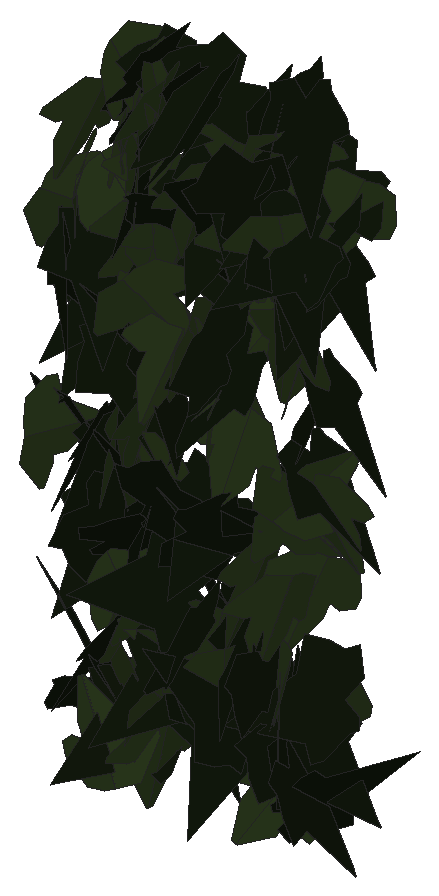
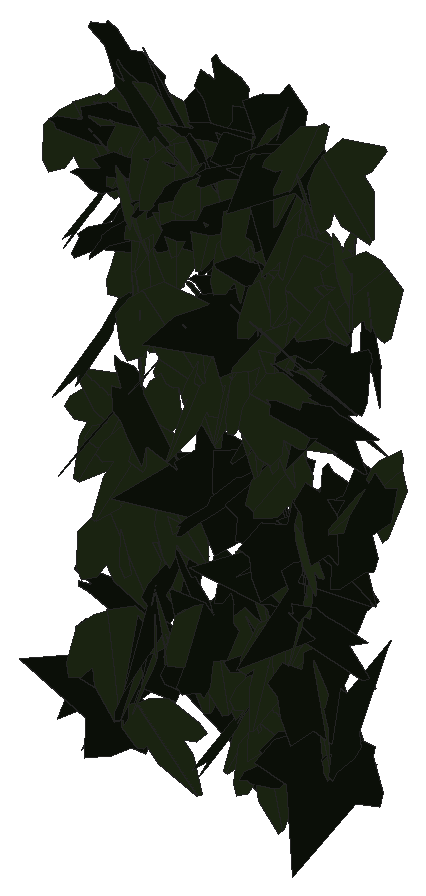
# SketchUp Ruby script. Lengths in inches.
U = 1.inch
M = Sketchup.active_model
def pt(a) = Geom::Point3d.new(a.map { |v| v * U })
def face(e, loops, mat)
  f = e.add_face(loops[0].map { |a| pt(a) })
  loops[1..].each { |l| e.add_face(l.map { |a| pt(a) }).erase! }
  f.material = f.back_material = mat if mat
  f
end
# faces: each face lists its corners as indices into pts; further lists are holes
def faces(e, pts, list, mat = nil) = list.each { |f| face(e, (f[0].is_a?(Array) ? f : [f]).map { |l| l.map { |i| pts[i] } }, mat) }
# xy, xz, yz: faces in a plane at the given z, y or x. An outline is a flat list of corners, or four numbers for a rectangle; further outlines are holes
def ring(l) = l.size == 4 ? [[l[0], l[1]], [l[2], l[1]], [l[2], l[3]], [l[0], l[3]]] : l.each_slice(2).to_a
def flat(e, list, mat, &to3) = list.each { |f| face(e, (f[0].is_a?(Array) ? f : [f]).map { |l| ring(l).map { |u, v| to3.(u, v) } }, mat) }
def xy(e, z, list, mat = nil) = flat(e, list, mat) { |x, y| [x, y, z] }
def xz(e, y, list, mat = nil) = flat(e, list, mat) { |x, z| [x, y, z] }
def yz(e, x, list, mat = nil) = flat(e, list, mat) { |y, z| [x, y, z] }
def lines(e, pts, list) = list.each { |a, b| e.add_line(pt(pts[a]), pt(pts[b])) }
# prism: a flat outline (further loops are holes) pulled along v
def prism(e, loops, v, mat = nil)
  f = face(e, loops, mat); d = Geom::Vector3d.new(v.map { |x| x * U })
  f.pushpull(f.normal.samedirection?(d) ? d.length : -d.length)
end
def box(e, o, s, mat = nil) = prism(e, [[o, [o[0] + s[0], o[1], o[2]], [o[0] + s[0], o[1] + s[1], o[2]], [o[0], o[1] + s[1], o[2]]]], [0, 0, s[2]], mat)
def at(x, y, z, deg = 0) = Geom::Transformation.translation(pt([x, y, z])) * Geom::Transformation.rotation(ORIGIN, Z_AXIS, deg.degrees)
def axes(o, x, y, z) = Geom::Transformation.new([*x, 0, *y, 0, *z, 0, *pt(o).to_a, 1])
def part(name) = M.definitions.add(name)
# library, detail: a bought-in or finely detailed component or shape, given as its bounding box
def library(name, o, s) = part(name).tap { |d| box(d.entities, o, s) }
def detail(e, o, s) = box(e.add_group.entities, o, s)
def put(e, d, t, mat = nil) = e.add_instance(d, t).tap { |i| i.material = mat if mat }
def group(e, t, mat = nil) = e.add_group.tap { |g| g.transformation = t; g.material = mat if mat }.entities
root = M.entities
M.materials.add("efeu1").color = [18, 25, 13]
M.materials.add("efeu2").color = [43, 57, 29]
c1 = part("ivyleaf_9")
p = [[1.54,2.16,1.25],[1.36,2.04,1.19],[-0.21,0.99,0.68],[-0.71,1.11,0.82],[-0.85,0.86,0.67],[-0.8,0.17,0.21],
  [-0.9,-0.01,0.1],[-0.67,-0.16,-0.02],[-0.08,-0.08,-0.05],[-0.03,-0.6,-0.4],[0.65,-0.88,-0.66],[0.83,-0.6,-0.49],
  [1.29,-0.42,-0.43],[1.8125,-0.07,-0.26],[1.21,0.44,0.15]]
faces(c1.entities,p,[[0,1,2,3,4,5,6,7,8,9,10,11,12,13,14]],"efeu1")
c2 = part("ivyleaf_10")
p = [[0,0.5,-0.03],[-0.0625,2.02,-0.43],[-0.19,2.01,-0.46],[-0.54,1.05,-0.29],[-0.52,0.625,-0.18],[-0.83,0.76,-0.28],
  [-1.16,0.64,-0.33],[-1.15,0.33,-0.24],[-0.77,-0.39,0.02],[-0.3,-0.51,0.16],[0.04,-0.48,0.23],[-0.02,2.01,-0.4375],
  [-0.06,2.01,-0.43],[0.04,-0.49,0.23],[0.67,-0.49,0.14],[1.38,0.36,-0.2],[1.375,0.51,-0.24],[0.81,0.65,-0.19],
  [0.62,0.59,-0.15],[0.6,1.09,-0.28],[0.5,1.23,-0.31]]
faces(c2.entities,p,[[0,1,2,3,4,5,6,7,8,9,10],[11,12,0,13,14,15,16,17,18,19,20]],"efeu2")
put(root,c1,axes([38.67,221.95,234.49],[0.02684,-0.49802,-0.03545],[0.01501,-0.03468,0.49857],[-0.49905,-0.02783,0.01309]))
put(root,c1,axes([37.72,221.7,236.9],[0.23111,-0.08001,0.43611],[0.40693,-0.157,-0.24445],[0.17605,0.46792,-0.00745]))
put(root,c1,axes([39.87,221.86,240.91],[-0.49337,0.01086,0.08043],[-0.08049,-0.0018,-0.49348],[-0.01043,-0.49988,0.00352]))
put(root,c2,axes([37.85,222.01,238.93],[-0.13592,-0.36457,0.31403],[0.09854,-0.3405,-0.35264],[0.47097,-0.03397,0.16441]))
put(root,c2,axes([37.17,221.69,233.48],[0.44407,0.09949,0.20712],[-0.20142,-0.04837,0.45507],[0.11059,-0.48761,-0.00288]))
put(root,c2,axes([37.52,221.63,241.15],[0.32751,-0.3069,-0.22034],[-0.07407,0.23379,-0.43572],[0.37048,0.31804,0.10767]))
put(root,c1,axes([38.39,221.43,235.41],[-0.09243,0.36788,0.32577],[-0.15461,0.29287,-0.37459],[-0.46642,-0.16998,0.05962]))
put(root,c2,axes([37.61,221.6,239.6],[-0.29405,-0.28547,-0.28643],[0.22578,0.17792,-0.40911],[0.3355,-0.36994,0.02427]))
put(root,c2,axes([37.58,221.89,238.06],[0.10743,-0.48116,0.0833],[0.01418,-0.08218,-0.493],[0.48812,0.10829,-0.00402]))
put(root,c1,axes([36.23,221.9375,239.73],[-0.14034,0.0231,-0.47934],[0.47476,-0.06621,-0.14219],[-0.07005,-0.49506,-0.00335]))
put(root,c2,axes([36.73,221.96,241.53],[-0.03882,-0.45261,0.2089],[-0.01385,-0.20847,-0.45426],[0.4983,-0.04105,0.00364]))
put(root,c1,axes([38.09,221.5,240.95],[0.38364,0.32065,0.00248],[0.002,0.00148,-0.49999],[-0.32066,0.38364,-0.00015]))
put(root,c2,axes([38.89,221.81,238.22],[0.49087,-0.006,-0.09491],[-0.09396,0.04644,-0.48889],[0.01469,0.4978,0.04447]))
put(root,c2,axes([36.34,221.45,237.46],[0.0512,-0.13144,-0.47969],[0.14467,0.46531,-0.11206],[0.47587,-0.12732,0.08568]))
put(root,c1,axes([39.7,221.7,234.26],[0.32273,-0.27841,-0.2614],[-0.18037,0.19055,-0.42563],[0.33662,0.36902,0.02256]))
put(root,c2,axes([39.52,221.77,240.93],[-0.40297,-0.29149,-0.05149],[0.04075,0.03153,-0.49734],[0.29318,-0.40502,-0.00166]))
put(root,c2,axes([37.52,221.82,237.43],[-0.41118,0.12215,-0.25692],[0.23899,-0.09665,-0.42842],[-0.15432,-0.47512,0.0211]))
put(root,c2,axes([38.97,222.05,236.5],[0.06527,-0.43435,0.23891],[0.06305,-0.23174,-0.43854],[0.4917,0.08738,0.02452]))
put(root,c2,axes([37.67,221.82,240.43],[-0.39272,-0.30944,0.0043],[-0.00512,-0.00045,-0.49997],[0.30943,-0.39274,-0.00281]))
put(root,c1,axes([38.66,221.78,239.08],[-0.37472,0.30294,0.13346],[-0.11842,0.06558,-0.48133],[-0.30913,-0.39234,0.0226]))
put(root,c1,axes([37.91,222.19,235.7],[-0.2392,-0.08834,0.4301],[-0.3403,-0.2722,-0.24516],[0.27745,-0.41001,0.07009]))
put(root,c2,axes([38.25,222,241.04],[-0.04847,-0.48874,0.09374],[-0.0001,-0.09417,-0.49105],[0.49764,-0.04763,0.00903]))
put(root,c1,axes([37.53,222.19,238.18],[0.10611,-0.39433,0.28853],[0.10101,-0.27117,-0.40775],[0.47806,0.14482,0.02211]))
put(root,c1,axes([39.39,222.0625,240.54],[0.11888,-0.48532,-0.01826],[-0.0035,0.01794,-0.49967],[0.48565,0.11893,0.00086]))
put(root,c1,axes([38.41,221.95,242.09],[-0.35969,0.30374,-0.16842],[0.10608,-0.1348,-0.46965],[-0.33071,-0.37359,0.03253]))
put(root,c1,axes([38.625,222.0625,234.43],[-0.44156,-0.15754,-0.1738],[0.16297,0.06042,-0.46882],[0.16871,-0.47067,-0.00201]))
put(root,c1,axes([38.25,222.29,236.89],[-0.1605,-0.41942,0.21983],[-0.01935,-0.22611,-0.44554],[0.47314,-0.15153,0.05635]))
put(root,c1,axes([36.72,222.13,239.7],[-0.04014,-0.49688,-0.0387],[0.00626,0.03832,-0.49849],[0.49835,-0.0405,0.00315]))
put(root,c1,axes([38.4,221.58,236.86],[0.06768,0.25198,-0.42653],[0.10725,0.41283,0.2609],[0.48365,-0.12681,0.00183]))
put(root,c2,axes([39.31,221.99,235.26],[0.33036,-0.37414,-0.02967],[-0.01675,0.02479,-0.4991],[0.37494,0.33076,0.00384]))
put(root,c1,axes([38.82,221.69,240.99],[0.02651,-0.00824,0.49923],[0.47113,0.16596,-0.02228],[-0.16534,0.47158,0.01656]))
put(root,c1,axes([38.67,222.12,238.9],[-0.46613,0.03952,-0.17653],[0.1672,-0.09216,-0.46212],[-0.06907,-0.48984,0.0727]))
put(root,c2,axes([39.27,222.08,236.19],[-0.14128,-0.4588,0.1398],[-0.00131,-0.14537,-0.4784],[0.47962,-0.13554,0.03987]))
put(root,c1,axes([37.33,222.31,233.92],[-0.28777,-0.29923,0.27867],[-0.20162,-0.19261,-0.41503],[0.35572,-0.35123,-0.00981]))
put(root,c2,axes([36.29,222.3,240.32],[-0.018,-0.10508,-0.4885],[0.17105,-0.46058,0.09277],[-0.46948,-0.16378,0.05253]))
put(root,c1,axes([37.9375,222.22,234.75],[-0.44206,-0.19184,0.13332],[-0.11922,-0.06015,-0.48184],[0.20091,-0.4578,0.00744]))
put(root,c2,axes([38.53,221.97,235.1],[-0.24749,-0.43359,-0.0274],[0.01612,0.02234,-0.49924],[0.43415,-0.24799,0.00292]))
put(root,c2,axes([37.62,222.06,233.88],[-0.12591,-0.48187,0.04418],[-0.00573,-0.04416,-0.49801],[0.48385,-0.12592,0.0056]))
put(root,c1,axes([36.67,221.82,239.13],[0.46715,0.0236,-0.17666],[-0.17752,0.01719,-0.46711],[-0.01598,0.49915,0.02444]))
put(root,c1,axes([37.11,222.08,238.58],[0.04891,-0.46912,-0.16595],[-0.00424,0.16635,-0.4715],[0.49758,0.04753,0.0123]))
put(root,c1,axes([40.03,222.1,235.12],[-0.43837,0.11295,0.2123],[-0.21653,0.00665,-0.45063],[-0.10463,-0.48703,0.04308]))
put(root,c1,axes([39.11,221.79,235.48],[0.1381,-0.18588,-0.44315],[-0.27503,0.34753,-0.23148],[0.39407,0.30769,-0.00626]))
put(root,c1,axes([37.43,222.3,241.14],[-0.13396,0.08362,-0.47441],[0.34041,-0.33198,-0.15463],[-0.34085,-0.36441,0.03201]))
put(root,c1,axes([38.6,222.18,235.73],[-0.34743,0.01009,-0.35944],[0.35899,-0.01885,-0.34752],[-0.02057,-0.49954,0.00586]))
put(root,c2,axes([39.47,221.96,239.45],[-0.46317,0.04588,0.18268],[-0.18294,0.00583,-0.46529],[-0.04483,-0.49786,0.01139]))
put(root,c1,axes([37.02,222.12,235.05],[-0.24673,0.33892,-0.2725],[0.09087,-0.26621,-0.41337],[-0.42528,-0.25351,0.06977]))
put(root,c2,axes([39.12,222.28,234.66],[-0.08062,0.28408,-0.40348],[0.13307,-0.38117,-0.29496],[-0.47518,-0.15494,-0.01415]))
put(root,c2,axes([39.35,221.93,240.52],[-0.05029,-0.44461,-0.22315],[0.05058,0.21856,-0.44685],[0.49489,-0.06751,0.02299]))
put(root,c1,axes([40.08,222.02,240.8125],[-0.4043,0.25445,0.14764],[-0.13008,0.07045,-0.47762],[-0.26386,-0.42461,0.00923]))
put(root,c2,axes([37.61,222.17,240.85],[-0.3513,-0.3026,0.18714],[-0.10735,-0.16059,-0.46118],[0.33921,-0.36421,0.04786]))
put(root,c1,axes([36.97,222.24,236.05],[-0.02743,0.15334,0.47512],[0.1272,-0.45798,0.15515],[0.48277,0.12938,-0.01389]))
put(root,c2,axes([37.82,222.15,240.3],[-0.18278,-0.46164,0.05898],[-0.01094,-0.05908,-0.49638],[0.46526,-0.18275,0.0115]))
put(root,c2,axes([37.53,222.08,241.8],[0.02535,-0.49402,-0.07282],[-0.01083,0.07235,-0.49462],[0.49924,0.02665,-0.00703]))
put(root,c1,axes([39.45,222.24,242.28],[-0.28256,-0.14245,-0.38713],[0.38394,0.08077,-0.30995],[0.15084,-0.47242,0.06374]))
put(root,c2,axes([37.05,222.18,241.44],[0.33291,-0.3728,0.01399],[0.00764,-0.01193,-0.4998],[0.37298,0.33299,-0.00224]))
put(root,c1,axes([37.03,221.86,236.15],[0.32897,-0.05469,0.37254],[0.35815,0.19812,-0.28718],[-0.11621,0.4558,0.16952]))
put(root,c1,axes([39.5,221.94,234.57],[-0.06931,-0.1501,-0.47188],[0.1604,0.44398,-0.16478],[0.46847,-0.17422,-0.01339]))
put(root,c2,axes([37.09,221.97,234.74],[-0.30622,0.15199,0.36487],[-0.35572,0.09524,-0.33822],[-0.17231,-0.46672,0.04981]))
put(root,c2,axes([39.46,221.97,237.34],[-0.22418,-0.29717,0.33382],[0.18247,0.28006,0.37185],[-0.40798,0.28855,-0.01712]))
put(root,c2,axes([37.69,221.89,234.46],[-0.13567,-0.3283,-0.35187],[0.11903,0.33133,-0.35504],[0.46629,-0.1801,-0.01175]))
put(root,c2,axes([36.29,221.88,240.24],[-0.16679,-0.21649,-0.41871],[0.28532,0.30717,-0.27247],[0.3752,-0.32982,0.02107]))
put(root,c1,axes([36.5,222.26,234.35],[0.21962,-0.39446,0.21486],[-0.09759,0.19155,0.45143],[-0.43845,-0.24022,0.00714]))
put(root,c2,axes([37.05,221.97,235.71],[0.08329,0.46417,0.16616],[0.03323,0.16284,-0.47157],[-0.49189,0.0896,-0.00372]))
put(root,c2,axes([39.17,222.19,233.75],[0.43984,-0.00955,-0.2376],[-0.23703,0.02239,-0.43968],[0.01904,0.49941,0.01516]))
put(root,c1,axes([36.04,222.23,237.25],[0.33245,-0.21457,0.30567],[0.26296,-0.15611,-0.39558],[0.2652,0.42378,0.00905]))
put(root,c1,axes([39.52,222.01,233.97],[-0.03799,-0.29274,0.40356],[0.11277,0.3892,0.29293],[-0.48563,0.11327,0.03645]))
put(root,c1,axes([39.66,221.86,233.71],[0.14021,0.41699,-0.23761],[0.03991,0.23656,0.43869],[0.47828,-0.14198,0.03305]))
put(root,c2,axes([38.44,222.2,241.32],[-0.43425,-0.133,0.20913],[-0.18799,-0.09818,-0.45279],[0.16151,-0.47188,0.03527]))
put(root,c1,axes([36.68,222.23,237.5],[-0.26436,0.34244,-0.2507],[0.1643,-0.18975,-0.43244],[-0.39131,-0.31101,-0.0122]))
put(root,c1,axes([37.91,222.45,240.01],[-0.44141,-0.20088,0.12166],[-0.10556,-0.06166,-0.48482],[0.20979,-0.4537,0.01202]))
put(root,c2,axes([37.8,222.16,234.63],[0.19847,0.00403,-0.45891],[-0.44735,0.11327,-0.19248],[0.10241,0.48698,0.04856]))
put(root,c2,axes([38.83,222.1875,240.5],[-0.39645,-0.30432,0.01469],[-0.01138,-0.0093,-0.49978],[0.30446,-0.39662,0.00045]))
put(root,c1,axes([38.64,222.14,241.2],[-0.24612,0.32126,0.29363],[0.15082,-0.25347,0.40374],[0.40826,0.28731,0.02787]))
put(root,c2,axes([38.21,222.15,240.98],[-0.24478,-0.41241,-0.14143],[0.09554,0.10751,-0.47887],[0.42539,-0.26145,0.02617]))
put(root,c2,axes([37.43,222.31,236.23],[0.4689,-0.12114,0.12432],[0.12147,-0.0268,-0.48428],[0.12399,0.48436,0.00429]))
put(root,c1,axes([39.4375,222.53,240.22],[-0.19535,-0.45639,0.05953],[-0.01774,-0.05716,-0.49641],[0.45992,-0.19606,0.00614]))
put(root,c2,axes([37.35,222.24,239.86],[-0.15481,-0.47261,-0.05172],[0.0352,0.04286,-0.49691],[0.47412,-0.1575,0.02]))
put(root,c1,axes([38.34,222.47,241.17],[-0.04719,-0.49766,-0.01017],[-0.00904,0.01107,-0.4998],[0.49769,-0.04698,-0.01004]))
put(root,c2,axes([37.6875,222.26,238.57],[-0.0072,-0.49654,-0.05824],[0.00598,0.05816,-0.49657],[0.49991,-0.00785,0.0051]))
put(root,c2,axes([40.01,222.41,241.24],[-0.34873,-0.28414,0.2183],[-0.09449,-0.22092,-0.43848],[0.34563,-0.34708,0.10039]))
put(root,c2,axes([39.68,222.21,237.52],[-0.46461,0.05174,-0.17737],[0.17614,-0.02093,-0.46748],[-0.0558,-0.49687,0.00122]))
put(root,c2,axes([37.25,222.21,239.36],[0.09019,0.49179,0.00262],[0.00038,0.0026,-0.49999],[-0.4918,0.09019,0.00009]))
put(root,c2,axes([38.21,222.31,235.34],[-0.41841,-0.24357,0.12492],[-0.11532,-0.05008,-0.48393],[0.24826,-0.43378,-0.01427]))
put(root,c2,axes([38.48,222.08,238.35],[0.0591,-0.36551,-0.33603],[0.09439,0.3405,-0.35377],[0.48744,-0.02162,0.10924]))
put(root,c1,axes([38.15,222.61,241.9],[-0.4663,-0.16594,0.07094],[-0.01701,-0.15525,-0.47498],[0.17966,-0.44538,0.13914]))
put(root,c1,axes([38.18,222.58,240.69],[-0.2667,-0.42292,0.00255],[0.00035,-0.00324,-0.49999],[0.42293,-0.26669,0.00203]))
put(root,c1,axes([37.54,222.0625,241.75],[0.02392,0.49917,0.01612],[0.00117,0.01608,-0.49974],[-0.49943,0.02395,-0.0004]))
put(root,c1,axes([39.8125,222.56,241.4],[-0.4347,-0.24382,0.03982],[-0.03549,-0.01813,-0.49841],[0.24449,-0.43615,-0.00154]))
put(root,c2,axes([39.3,222.14,237.23],[-0.18577,-0.34522,-0.31035],[0.20185,0.24095,-0.38885],[0.41803,-0.26976,0.04984]))
put(root,c1,axes([39.65,222.45,240.5],[0.23853,-0.43944,-0.00111],[-0.00403,-0.00092,-0.49998],[0.43942,0.23853,-0.00398]))
put(root,c1,axes([36.89,222.55,237.17],[0.00754,0.18312,-0.4652],[0.01278,-0.46517,-0.1829],[-0.49978,-0.00913,-0.0117]))
put(root,c2,axes([39.1875,222.24,241.64],[-0.44352,-0.16619,-0.16022],[0.14397,0.07214,-0.47336],[0.18045,-0.46602,-0.01614]))
put(root,c2,axes([37.37,222.25,241.94],[-0.1281,0.48305,0.01591],[-0.01109,0.01352,-0.49969],[-0.48318,-0.12837,0.00725]))
put(root,c2,axes([37.91,222.17,238.87],[0.08796,-0.40248,-0.28333],[0.0553,0.29407,-0.40058],[0.48909,0.03913,0.09625]))
put(root,c2,axes([36.82,222.17,240.52],[0.21618,0.38509,0.23446],[0.11869,0.20224,-0.4416],[-0.43495,0.24658,-0.00397]))
put(root,c1,axes([39.1,222.64,240.45],[-0.04653,-0.48782,0.09932],[0.00543,-0.10025,-0.48982],[0.4978,-0.04451,0.01463]))
put(root,c1,axes([37.5,222.29,239.35],[-0.34465,0.2786,0.2315],[-0.23009,0.07842,-0.43693],[-0.27977,-0.40771,0.07415]))
put(root,c1,axes([37.69,222.46,234.39],[0.26118,-0.42614,-0.0139],[-0.00672,0.01218,-0.49981],[0.42631,0.26126,0.00063]))
put(root,c1,axes([36.61,222.1,234.17],[0.28353,0.41001,-0.03871],[-0.02722,-0.02824,-0.49846],[-0.41094,0.28477,0.0063]))
put(root,c1,axes([39.47,222.34,237.83],[0.27861,-0.37964,-0.16807],[-0.05466,0.16711,-0.46807],[0.41157,0.27919,0.05162]))
put(root,c2,axes([37.125,222.625,238.68],[-0.16504,-0.21221,0.42158],[-0.22317,-0.35845,-0.26779],[0.41588,-0.27656,0.0236]))
put(root,c2,axes([39.61,222.4,234.79],[-0.25965,-0.42618,0.0309],[-0.01499,-0.02705,-0.49904],[0.42703,-0.26008,0.00127]))
put(root,c2,axes([39.36,222.22,239.16],[0.18141,-0.34066,-0.31787],[-0.12881,0.29115,-0.38553],[0.44777,0.22177,0.01787]))
put(root,c2,axes([37.14,222.38,240.2],[0.2738,-0.01122,-0.41822],[-0.41272,0.07464,-0.2722],[0.06854,0.49427,0.03161]))
put(root,c2,axes([36.95,222.4,241.02],[-0.10564,0.47676,-0.10745],[0.00524,-0.10882,-0.48799],[-0.48868,-0.10423,0.01799]))
put(root,c2,axes([37.32,222.27,235.43],[-0.09212,-0.44169,-0.21546],[0.07851,0.20317,-0.45006],[0.48513,-0.11676,0.03192]))
put(root,c1,axes([36.74,222.57,239.13],[-0.49769,-0.00925,-0.04714],[0.04786,-0.05354,-0.49482],[0.00411,-0.49704,0.05418]))
put(root,c2,axes([36.6,222.64,237.22],[0.20347,-0.34331,0.30123],[0.1686,-0.25002,-0.39883],[0.42447,0.26387,0.01402]))
put(root,c1,axes([36.75,222.6,236.09],[-0.47866,-0.13727,-0.04517],[0.04889,-0.00675,-0.49756],[0.13599,-0.48074,0.01988]))
put(root,c2,axes([39.4,222.56,236.27],[-0.32022,-0.32996,0.19642],[-0.08407,-0.1893,-0.45508],[0.37468,-0.32448,0.06576]))
put(root,c1,axes([37.51,222.77,241.76],[-0.2726,-0.4042,0.11095],[0.01334,-0.14065,-0.47962],[0.41894,-0.25853,0.08747]))
put(root,c2,axes([36.92,222.22,241.97],[-0.0415,0.46022,0.191],[-0.02882,0.18912,-0.46196],[-0.49744,-0.04935,0.01083]))
put(root,c1,axes([36.61,222.09,236.32],[0.04345,-0.00652,-0.49807],[-0.08313,0.49285,-0.0137],[0.49112,0.084,0.04174]))
put(root,c1,axes([39.41,222.71,240.98],[-0.44249,-0.18255,0.14449],[-0.10956,-0.11053,-0.47516],[0.20542,-0.45217,0.05782]))
put(root,c2,axes([39.26,222.55,240.9],[0.21061,-0.44974,0.05814],[0.01914,-0.05523,-0.49657],[0.45308,0.21139,-0.00605]))
put(root,c1,axes([37.18,222.03,241.85],[0.14585,0.34462,0.33161],[0.12029,0.30911,-0.37414],[-0.46288,0.18892,0.00726]))
put(root,c1,axes([39.23,222.62,238.14],[-0.35319,0.1696,-0.31063],[0.25176,-0.18804,-0.38892],[-0.24874,-0.43113,0.04744]))
put(root,c1,axes([39.53,222.49,238.81],[0.32214,-0.37178,-0.08948],[-0.05789,0.06824,-0.49193],[0.37798,0.3273,0.00092]))
put(root,c1,axes([39.22,222.55,242.04],[-0.42793,0.22029,-0.13544],[0.10789,-0.08589,-0.48061],[-0.23501,-0.44056,0.02597]))
put(root,c2,axes([38.61,222.47,241.1875],[-0.13209,-0.4794,-0.05225],[0.02524,0.04723,-0.49712],[0.48157,-0.13397,0.01172]))
put(root,c2,axes([38.83,222.52,241.32],[-0.05729,-0.4967,0.00234],[-0.00137,-0.0022,-0.49999],[0.49671,-0.05729,-0.0011]))
put(root,c1,axes([37.9,222.72,235.22],[0.13014,-0.21564,0.43193],[0.23447,-0.36281,-0.25178],[0.422,0.26808,0.00669]))
put(root,c2,axes([38.83,222.61,239.3125],[-0.37526,-0.15402,0.29233],[-0.21242,-0.22639,-0.39195],[0.2531,-0.41836,0.10448]))
put(root,c2,axes([36.89,222.36,236.45],[-0.4014,0.27996,0.10247],[-0.08723,0.05405,-0.48936],[-0.28508,-0.41073,0.00545]))
put(root,c1,axes([37.67,222.4375,239.63],[0.44446,-0.13503,0.18499],[0.17398,-0.06358,-0.46442],[0.14894,0.47721,-0.00953]))
put(root,c1,axes([36.57,222.71,238.84],[-0.44285,-0.21229,-0.09389],[0.10577,-0.00452,-0.48866],[0.20662,-0.45267,0.04891]))
